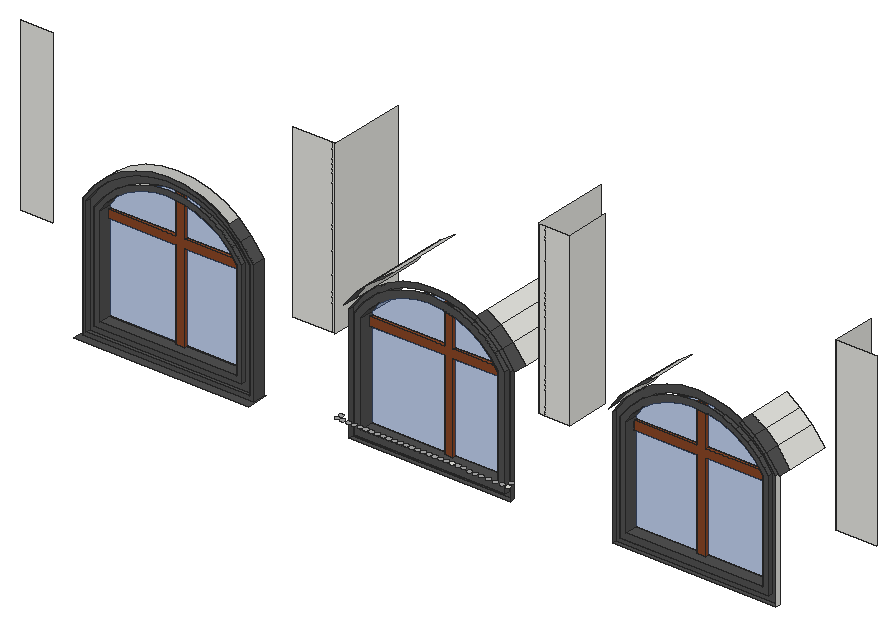
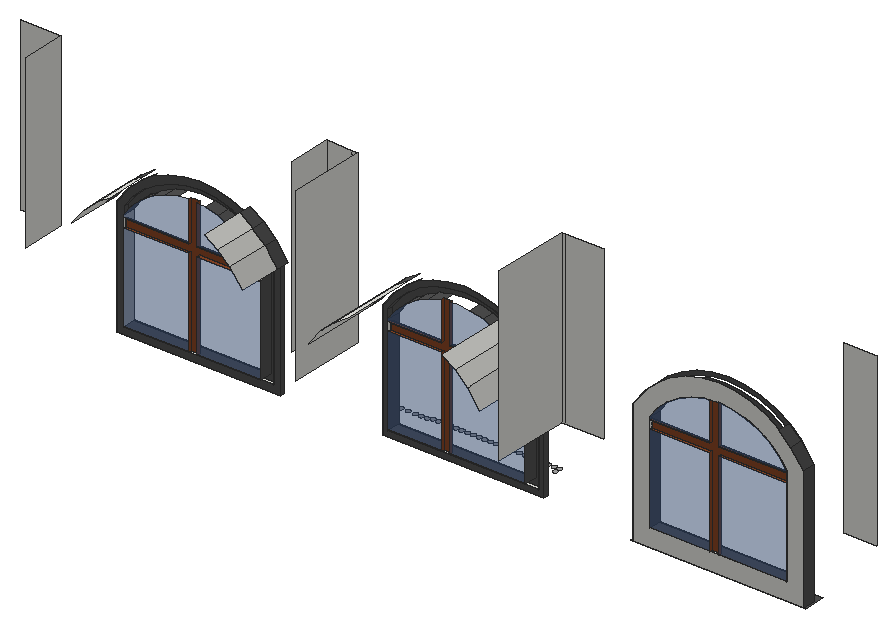
# SketchUp Ruby script. Lengths in inches.
U = 1.inch
M = Sketchup.active_model
def pt(a) = Geom::Point3d.new(a.map { |v| v * U })
def face(e, loops, mat)
  f = e.add_face(loops[0].map { |a| pt(a) })
  loops[1..].each { |l| e.add_face(l.map { |a| pt(a) }).erase! }
  f.material = f.back_material = mat if mat
  f
end
# faces: each face lists its corners as indices into pts; further lists are holes
def faces(e, pts, list, mat = nil) = list.each { |f| face(e, (f[0].is_a?(Array) ? f : [f]).map { |l| l.map { |i| pts[i] } }, mat) }
# xy, xz, yz: faces in a plane at the given z, y or x. An outline is a flat list of corners, or four numbers for a rectangle; further outlines are holes
def ring(l) = l.size == 4 ? [[l[0], l[1]], [l[2], l[1]], [l[2], l[3]], [l[0], l[3]]] : l.each_slice(2).to_a
def flat(e, list, mat, &to3) = list.each { |f| face(e, (f[0].is_a?(Array) ? f : [f]).map { |l| ring(l).map { |u, v| to3.(u, v) } }, mat) }
def xy(e, z, list, mat = nil) = flat(e, list, mat) { |x, y| [x, y, z] }
def xz(e, y, list, mat = nil) = flat(e, list, mat) { |x, z| [x, y, z] }
def yz(e, x, list, mat = nil) = flat(e, list, mat) { |y, z| [x, y, z] }
def lines(e, pts, list) = list.each { |a, b| e.add_line(pt(pts[a]), pt(pts[b])) }
# prism: a flat outline (further loops are holes) pulled along v
def prism(e, loops, v, mat = nil)
  f = face(e, loops, mat); d = Geom::Vector3d.new(v.map { |x| x * U })
  f.pushpull(f.normal.samedirection?(d) ? d.length : -d.length)
end
def box(e, o, s, mat = nil) = prism(e, [[o, [o[0] + s[0], o[1], o[2]], [o[0] + s[0], o[1] + s[1], o[2]], [o[0], o[1] + s[1], o[2]]]], [0, 0, s[2]], mat)
def at(x, y, z, deg = 0) = Geom::Transformation.translation(pt([x, y, z])) * Geom::Transformation.rotation(ORIGIN, Z_AXIS, deg.degrees)
def axes(o, x, y, z) = Geom::Transformation.new([*x, 0, *y, 0, *z, 0, *pt(o).to_a, 1])
def part(name) = M.definitions.add(name)
# library, detail: a bought-in or finely detailed component or shape, given as its bounding box
def library(name, o, s) = part(name).tap { |d| box(d.entities, o, s) }
def detail(e, o, s) = box(e.add_group.entities, o, s)
def put(e, d, t, mat = nil) = e.add_instance(d, t).tap { |i| i.material = mat if mat }
def group(e, t, mat = nil) = e.add_group.tap { |g| g.transformation = t; g.material = mat if mat }.entities
root = M.entities
M.materials.add("[0042_Sienna]").color = [137, 70, 38]
M.materials.add("[0132_LightGray]").color = [169, 169, 169]
M.materials.add("[0135_DarkGray]").color = [81, 81, 81]
M.materials.add("[Translucent Glass Blue]").color = [66, 99, 158]
M.materials["[Translucent Glass Blue]"].alpha = 0.5
xy(root,182.98,[[429.64,40.6875,544.9375,43.6875]],"[0135_DarkGray]")
xy(root,183.1,[[55.95,40.6875,176.64,49.6875]])
xy(root,183.1,[[54.57,34.6875,177.76,34.6875,177.76,49.6875,176.64,49.6875,176.64,40.6875,55.95,40.6875,55.95,49.6875,54.57,49.6875]],"[0135_DarkGray]")
xy(root,183.73,[[243.9,40.6875,357.68,43.6875]],"[0135_DarkGray]")
xy(root,185.78,[[58.63,40.6875,173.95,43.6875]],"[0135_DarkGray]")
xy(root,187.34,[[247.51,40.6875,354.08,43.6875]])
xy(root,188.0625,[[434.73,40.6875,539.86,43.6875]])
xy(root,191.43,[[64.29,40.6875,168.3,43.6875]],"[0135_DarkGray]")
xy(root,192.28,[[305.64,47.6875,311.64,49.6875],[483.7,47.6875,489.7,49.6875]])
xy(root,192.28,[[252.45,40.6875,349.14,40.6875,349.14,49.6875,311.64,49.6875,311.64,47.6875,305.64,47.6875,305.64,49.6875,252.45,49.6875],[438.95,40.6875,535.64,40.6875,535.64,49.6875,489.7,49.6875,489.7,47.6875,483.7,47.6875,483.7,49.6875,438.95,49.6875]],"[0135_DarkGray]")
xy(root,195.1,[[116.29,47.6875,122.29,49.6875]])
xy(root,195.1,[[67.95,40.6875,164.64,40.6875,164.64,49.6875,122.29,49.6875,122.29,47.6875,116.29,47.6875,116.29,49.6875,67.95,49.6875]],"[0135_DarkGray]")
xy(root,197.66,[[361.68,32.09,362.06,32.13,362.4,32.28,362.7,32.51,362.93,32.8,363.07,33.15,363.12,33.52,363.07,33.89,362.93,34.24,362.7,34.54,362.4,34.77,362.06,34.91,361.68,34.96,361.3125,34.91,360.97,34.77,360.67,34.54,360.4375,34.24,360.3,33.89,360.25,33.52,360.3,33.15,360.4375,32.8,360.67,32.51,360.97,32.28,361.3125,32.13]])
xy(root,197.66,[[334.56,32.09,334.93,32.13,335.28,32.28,335.58,32.51,335.8,32.8,335.95,33.15,336,33.52,335.95,33.89,335.8,34.24,335.58,34.54,335.28,34.77,334.93,34.91,334.56,34.96,334.1875,34.91,333.84,34.77,333.54,34.54,333.3125,34.24,333.17,33.89,333.12,33.52,333.17,33.15,333.3125,32.8,333.54,32.51,333.84,32.28,334.1875,32.13],[338.62,32.09,338.99,32.13,339.34,32.28,339.64,32.51,339.87,32.8,340.01,33.15,340.06,33.52,340.01,33.89,339.87,34.24,339.64,34.54,339.34,34.77,338.99,34.91,338.62,34.96,338.25,34.91,337.9,34.77,337.6,34.54,337.375,34.24,337.23,33.89,337.18,33.52,337.23,33.15,337.375,32.8,337.6,32.51,337.9,32.28,338.25,32.13],[342.68,32.09,343.06,32.13,343.4,32.28,343.7,32.51,343.93,32.8,344.07,33.15,344.12,33.52,344.07,33.89,343.93,34.24,343.7,34.54,343.4,34.77,343.06,34.91,342.68,34.96,342.3125,34.91,341.97,34.77,341.67,34.54,341.4375,34.24,341.3,33.89,341.25,33.52,341.3,33.15,341.4375,32.8,341.67,32.51,341.97,32.28,342.3125,32.13],[347.93,32.09,348.31,32.13,348.65,32.28,348.95,32.51,349.18,32.8,349.32,33.15,349.37,33.52,349.32,33.89,349.18,34.24,348.95,34.54,348.65,34.77,348.31,34.91,347.93,34.96,347.5625,34.91,347.22,34.77,346.92,34.54,346.6875,34.24,346.55,33.89,346.5,33.52,346.55,33.15,346.6875,32.8,346.92,32.51,347.22,32.28,347.5625,32.13],[352.81,32.09,353.18,32.13,353.53,32.28,353.83,32.51,354.05,32.8,354.2,33.15,354.25,33.52,354.2,33.89,354.05,34.24,353.83,34.54,353.53,34.77,353.18,34.91,352.81,34.96,352.4375,34.91,352.09,34.77,351.79,34.54,351.5625,34.24,351.42,33.89,351.37,33.52,351.42,33.15,351.5625,32.8,351.79,32.51,352.09,32.28,352.4375,32.13],
  [357.56,32.09,357.93,32.13,358.28,32.28,358.58,32.51,358.8,32.8,358.95,33.15,359,33.52,358.95,33.89,358.8,34.24,358.58,34.54,358.28,34.77,357.93,34.91,357.56,34.96,357.1875,34.91,356.84,34.77,356.54,34.54,356.3125,34.24,356.17,33.89,356.12,33.52,356.17,33.15,356.3125,32.8,356.54,32.51,356.84,32.28,357.1875,32.13],[360.7,36.35,361.07,36.4,361.41,36.54,361.71,36.77,361.94,37.07,362.08,37.41,362.13,37.78,362.08,38.16,361.94,38.5,361.71,38.8,361.41,39.03,361.07,39.17,360.7,39.22,360.32,39.17,359.98,39.03,359.68,38.8,359.45,38.5,359.31,38.16,359.26,37.78,359.31,37.41,359.45,37.07,359.68,36.77,359.98,36.54,360.32,36.4]],"[0132_LightGray]")
xy(root,198.6,[[322.37,32.09,322.74,32.13,323.09,32.28,323.39,32.51,323.62,32.8,323.76,33.15,323.81,33.52,323.76,33.89,323.62,34.24,323.39,34.54,323.09,34.77,322.74,34.91,322.37,34.96,322,34.91,321.65,34.77,321.35,34.54,321.125,34.24,320.98,33.89,320.93,33.52,320.98,33.15,321.125,32.8,321.35,32.51,321.65,32.28,322,32.13]])
xy(root,198.6,[[241.12,32.09,241.49,32.13,241.84,32.28,242.14,32.51,242.37,32.8,242.51,33.15,242.56,33.52,242.51,33.89,242.37,34.24,242.14,34.54,241.84,34.77,241.49,34.91,241.12,34.96,240.75,34.91,240.4,34.77,240.1,34.54,239.875,34.24,239.73,33.89,239.68,33.52,239.73,33.15,239.875,32.8,240.1,32.51,240.4,32.28,240.75,32.13],[245.18,32.09,245.56,32.13,245.9,32.28,246.2,32.51,246.43,32.8,246.57,33.15,246.62,33.52,246.57,33.89,246.43,34.24,246.2,34.54,245.9,34.77,245.56,34.91,245.18,34.96,244.8125,34.91,244.47,34.77,244.17,34.54,243.9375,34.24,243.8,33.89,243.75,33.52,243.8,33.15,243.9375,32.8,244.17,32.51,244.47,32.28,244.8125,32.13],[249.25,32.09,249.62,32.13,249.97,32.28,250.26,32.51,250.49,32.8,250.63,33.15,250.68,33.52,250.63,33.89,250.49,34.24,250.26,34.54,249.97,34.77,249.62,34.91,249.25,34.96,248.875,34.91,248.53,34.77,248.23,34.54,248,34.24,247.86,33.89,247.81,33.52,247.86,33.15,248,32.8,248.23,32.51,248.53,32.28,248.875,32.13],[253.31,32.09,253.68,32.13,254.03,32.28,254.33,32.51,254.55,32.8,254.7,33.15,254.75,33.52,254.7,33.89,254.55,34.24,254.33,34.54,254.03,34.77,253.68,34.91,253.31,34.96,252.9375,34.91,252.59,34.77,252.29,34.54,252.0625,34.24,251.92,33.89,251.87,33.52,251.92,33.15,252.0625,32.8,252.29,32.51,252.59,32.28,252.9375,32.13],[257.37,32.09,257.74,32.13,258.09,32.28,258.39,32.51,258.62,32.8,258.76,33.15,258.81,33.52,258.76,33.89,258.62,34.24,258.39,34.54,258.09,34.77,257.74,34.91,257.37,34.96,257,34.91,256.65,34.77,256.35,34.54,256.125,34.24,255.98,33.89,255.93,33.52,255.98,33.15,256.125,32.8,256.35,32.51,256.65,32.28,257,32.13],
  [261.43,32.09,261.81,32.13,262.15,32.28,262.45,32.51,262.68,32.8,262.82,33.15,262.87,33.52,262.82,33.89,262.68,34.24,262.45,34.54,262.15,34.77,261.81,34.91,261.43,34.96,261.0625,34.91,260.72,34.77,260.42,34.54,260.1875,34.24,260.05,33.89,260,33.52,260.05,33.15,260.1875,32.8,260.42,32.51,260.72,32.28,261.0625,32.13],[265.5,32.09,265.87,32.13,266.22,32.28,266.51,32.51,266.74,32.8,266.88,33.15,266.93,33.52,266.88,33.89,266.74,34.24,266.51,34.54,266.22,34.77,265.87,34.91,265.5,34.96,265.125,34.91,264.78,34.77,264.48,34.54,264.25,34.24,264.11,33.89,264.06,33.52,264.11,33.15,264.25,32.8,264.48,32.51,264.78,32.28,265.125,32.13],[269.56,32.09,269.93,32.13,270.28,32.28,270.58,32.51,270.8,32.8,270.95,33.15,271,33.52,270.95,33.89,270.8,34.24,270.58,34.54,270.28,34.77,269.93,34.91,269.56,34.96,269.1875,34.91,268.84,34.77,268.54,34.54,268.3125,34.24,268.17,33.89,268.12,33.52,268.17,33.15,268.3125,32.8,268.54,32.51,268.84,32.28,269.1875,32.13],[273.62,32.09,273.99,32.13,274.34,32.28,274.64,32.51,274.87,32.8,275.01,33.15,275.06,33.52,275.01,33.89,274.87,34.24,274.64,34.54,274.34,34.77,273.99,34.91,273.62,34.96,273.25,34.91,272.9,34.77,272.6,34.54,272.375,34.24,272.23,33.89,272.18,33.52,272.23,33.15,272.375,32.8,272.6,32.51,272.9,32.28,273.25,32.13],[277.68,32.09,278.06,32.13,278.4,32.28,278.7,32.51,278.93,32.8,279.07,33.15,279.12,33.52,279.07,33.89,278.93,34.24,278.7,34.54,278.4,34.77,278.06,34.91,277.68,34.96,277.3125,34.91,276.97,34.77,276.67,34.54,276.4375,34.24,276.3,33.89,276.25,33.52,276.3,33.15,276.4375,32.8,276.67,32.51,276.97,32.28,277.3125,32.13],
  [281.75,32.09,282.12,32.13,282.47,32.28,282.76,32.51,282.99,32.8,283.13,33.15,283.18,33.52,283.13,33.89,282.99,34.24,282.76,34.54,282.47,34.77,282.12,34.91,281.75,34.96,281.375,34.91,281.03,34.77,280.73,34.54,280.5,34.24,280.36,33.89,280.31,33.52,280.36,33.15,280.5,32.8,280.73,32.51,281.03,32.28,281.375,32.13],[285.81,32.09,286.18,32.13,286.53,32.28,286.83,32.51,287.05,32.8,287.2,33.15,287.25,33.52,287.2,33.89,287.05,34.24,286.83,34.54,286.53,34.77,286.18,34.91,285.81,34.96,285.4375,34.91,285.09,34.77,284.79,34.54,284.5625,34.24,284.42,33.89,284.37,33.52,284.42,33.15,284.5625,32.8,284.79,32.51,285.09,32.28,285.4375,32.13],[289.87,32.09,290.24,32.13,290.59,32.28,290.89,32.51,291.12,32.8,291.26,33.15,291.31,33.52,291.26,33.89,291.12,34.24,290.89,34.54,290.59,34.77,290.24,34.91,289.87,34.96,289.5,34.91,289.15,34.77,288.85,34.54,288.625,34.24,288.48,33.89,288.43,33.52,288.48,33.15,288.625,32.8,288.85,32.51,289.15,32.28,289.5,32.13],[293.93,32.09,294.31,32.13,294.65,32.28,294.95,32.51,295.18,32.8,295.32,33.15,295.37,33.52,295.32,33.89,295.18,34.24,294.95,34.54,294.65,34.77,294.31,34.91,293.93,34.96,293.5625,34.91,293.22,34.77,292.92,34.54,292.6875,34.24,292.55,33.89,292.5,33.52,292.55,33.15,292.6875,32.8,292.92,32.51,293.22,32.28,293.5625,32.13],[298,32.09,298.37,32.13,298.72,32.28,299.01,32.51,299.24,32.8,299.38,33.15,299.43,33.52,299.38,33.89,299.24,34.24,299.01,34.54,298.72,34.77,298.37,34.91,298,34.96,297.625,34.91,297.28,34.77,296.98,34.54,296.75,34.24,296.61,33.89,296.56,33.52,296.61,33.15,296.75,32.8,296.98,32.51,297.28,32.28,297.625,32.13],
  [302.06,32.09,302.43,32.13,302.78,32.28,303.08,32.51,303.3,32.8,303.45,33.15,303.5,33.52,303.45,33.89,303.3,34.24,303.08,34.54,302.78,34.77,302.43,34.91,302.06,34.96,301.6875,34.91,301.34,34.77,301.04,34.54,300.8125,34.24,300.67,33.89,300.62,33.52,300.67,33.15,300.8125,32.8,301.04,32.51,301.34,32.28,301.6875,32.13],[306.12,32.09,306.49,32.13,306.84,32.28,307.14,32.51,307.37,32.8,307.51,33.15,307.56,33.52,307.51,33.89,307.37,34.24,307.14,34.54,306.84,34.77,306.49,34.91,306.12,34.96,305.75,34.91,305.4,34.77,305.1,34.54,304.875,34.24,304.73,33.89,304.68,33.52,304.73,33.15,304.875,32.8,305.1,32.51,305.4,32.28,305.75,32.13],[310.18,32.09,310.56,32.13,310.9,32.28,311.2,32.51,311.43,32.8,311.57,33.15,311.62,33.52,311.57,33.89,311.43,34.24,311.2,34.54,310.9,34.77,310.56,34.91,310.18,34.96,309.8125,34.91,309.47,34.77,309.17,34.54,308.9375,34.24,308.8,33.89,308.75,33.52,308.8,33.15,308.9375,32.8,309.17,32.51,309.47,32.28,309.8125,32.13],[314.25,32.09,314.62,32.13,314.97,32.28,315.26,32.51,315.49,32.8,315.63,33.15,315.68,33.52,315.63,33.89,315.49,34.24,315.26,34.54,314.97,34.77,314.62,34.91,314.25,34.96,313.875,34.91,313.53,34.77,313.23,34.54,313,34.24,312.86,33.89,312.81,33.52,312.86,33.15,313,32.8,313.23,32.51,313.53,32.28,313.875,32.13],[318.31,32.09,318.68,32.13,319.03,32.28,319.33,32.51,319.55,32.8,319.7,33.15,319.75,33.52,319.7,33.89,319.55,34.24,319.33,34.54,319.03,34.77,318.68,34.91,318.31,34.96,317.9375,34.91,317.59,34.77,317.29,34.54,317.0625,34.24,316.92,33.89,316.87,33.52,316.92,33.15,317.0625,32.8,317.29,32.51,317.59,32.28,317.9375,32.13],
  [326.43,32.09,326.81,32.13,327.15,32.28,327.45,32.51,327.68,32.8,327.82,33.15,327.87,33.52,327.82,33.89,327.68,34.24,327.45,34.54,327.15,34.77,326.81,34.91,326.43,34.96,326.0625,34.91,325.72,34.77,325.42,34.54,325.1875,34.24,325.05,33.89,325,33.52,325.05,33.15,325.1875,32.8,325.42,32.51,325.72,32.28,326.0625,32.13],[330.5,32.09,330.87,32.13,331.22,32.28,331.51,32.51,331.74,32.8,331.88,33.15,331.93,33.52,331.88,33.89,331.74,34.24,331.51,34.54,331.22,34.77,330.87,34.91,330.5,34.96,330.125,34.91,329.78,34.77,329.48,34.54,329.25,34.24,329.11,33.89,329.06,33.52,329.11,33.15,329.25,32.8,329.48,32.51,329.78,32.28,330.125,32.13],[241.12,35.71,241.49,35.76,241.84,35.9,242.14,36.13,242.37,36.43,242.51,36.78,242.56,37.15,242.51,37.52,242.37,37.87,242.14,38.16,241.84,38.39,241.49,38.54,241.12,38.59,240.75,38.54,240.4,38.39,240.1,38.16,239.875,37.87,239.73,37.52,239.68,37.15,239.73,36.78,239.875,36.43,240.1,36.13,240.4,35.9,240.75,35.76]],"[0132_LightGray]")
xy(root,254.53,[[438.95,47.6875,483.7,49.6875],[489.7,47.6875,535.64,49.6875]],"[0042_Sienna]")
xy(root,254.85,[[252.45,47.6875,305.64,49.6875],[311.64,47.6875,349.14,49.6875]],"[0042_Sienna]")
xy(root,257.72,[[67.95,47.6875,116.29,49.6875],[122.29,47.6875,164.64,49.6875]],"[0042_Sienna]")
xy(root,260.53,[[438.95,47.6875,483.7,49.6875],[489.7,47.6875,535.64,49.6875]],"[0042_Sienna]")
xy(root,260.85,[[252.45,47.6875,305.64,49.6875],[311.64,47.6875,349.14,49.6875]],"[0042_Sienna]")
xy(root,263.72,[[67.95,47.6875,116.29,49.6875],[122.29,47.6875,164.64,49.6875]],"[0042_Sienna]")
xz(root,40.6875,[[[55.95,183.1,176.64,183.1,176.64,269.51,167.71,281.11,159.24,288.98,149.59,295.34,139.01,300.01,127.8125,302.86,116.29,303.82,104.77,302.86,93.57,300.01,83,295.34,73.34,288.98,64.875,281.11,55.95,269.51],[58.63,185.78,58.63,268.6,66.87,279.3,75.01,286.86,84.29,292.97,94.45,297.46,105.22,300.21,116.29,301.13,127.36,300.21,138.13,297.46,148.3,292.97,157.58,286.86,165.72,279.3,173.95,268.6,173.95,185.78]],[[247.51,187.34,354.08,187.34,354.08,264.3,346.97,273.53,339.37,280.6,330.7,286.31,321.2,290.5,311.14,293.07,300.79,293.93,290.44,293.07,280.38,290.5,270.89,286.31,262.22,280.6,254.61,273.53,247.51,264.3],[252.45,192.28,252.45,262.62,258.28,270.19,265.28,276.7,273.26,281.95,282,285.82,291.27,288.18,300.79,288.97,310.32,288.18,319.58,285.82,328.32,281.95,336.3,276.7,343.31,270.19,349.14,262.62,349.14,192.28]],[[434.73,188.0625,539.86,188.0625,539.86,264.05,532.9375,273.04,525.42,280.03,516.85,285.67,507.46,289.82,497.52,292.35,487.29,293.21,477.06,292.35,467.12,289.82,457.73,285.67,449.16,280.03,441.64,273.04,434.73,264.05],[438.95,192.28,438.95,262.62,444.78,270.19,451.78,276.7,459.76,281.95,468.5,285.82,477.77,288.18,487.29,288.97,496.82,288.18,506.08,285.82,514.82,281.95,522.8,276.7,529.81,270.19,535.64,262.62,535.64,192.28]],[[64.29,191.43,168.3,191.43,168.3,266.67,161.52,275.48,154.07,282.4,145.58,287.99,136.28,292.1,126.42,294.61,116.29,295.46,106.16,294.61,96.3,292.1,87,287.99,78.51,282.4,71.06,275.48,64.29,266.67],[67.95,195.1,67.95,265.43,73.78,273,80.78,279.51,88.76,284.77,97.5,288.63,106.77,290.99,116.29,291.78,125.82,290.99,135.08,288.63,143.82,284.77,151.8,279.51,158.81,273,164.64,265.43,164.64,195.1]]],"[0135_DarkGray]")
xz(root,43.6875,[[[429.64,182.98,544.9375,182.98,544.9375,265.78,536.71,276.48,528.57,284.04,519.29,290.15,509.13,294.64,498.36,297.38,487.29,298.31,476.22,297.38,465.45,294.64,455.29,290.15,446.01,284.04,437.875,276.48,429.64,265.78],[434.73,188.0625,434.73,264.05,441.64,273.04,449.16,280.03,457.73,285.67,467.12,289.82,477.06,292.35,487.29,293.21,497.52,292.35,507.46,289.82,516.85,285.67,525.42,280.03,532.9375,273.04,539.86,264.05,539.86,188.0625]],[[243.9,183.73,357.68,183.73,357.68,265.52,349.65,275.97,341.6,283.44,332.43,289.48,322.38,293.92,311.74,296.64,300.79,297.55,289.85,296.64,279.2,293.92,269.16,289.48,259.98,283.44,251.94,275.97,243.9,265.52],[247.51,187.34,247.51,264.3,254.61,273.53,262.22,280.6,270.89,286.31,280.38,290.5,290.44,293.07,300.79,293.93,311.14,293.07,321.2,290.5,330.7,286.31,339.37,280.6,346.97,273.53,354.08,264.3,354.08,187.34]],[[58.63,185.78,173.95,185.78,173.95,268.6,165.72,279.3,157.58,286.86,148.3,292.97,138.13,297.46,127.36,300.21,116.29,301.13,105.22,300.21,94.45,297.46,84.29,292.97,75.01,286.86,66.87,279.3,58.63,268.6],[64.29,191.43,64.29,266.67,71.06,275.48,78.51,282.4,87,287.99,96.3,292.1,106.16,294.61,116.29,295.46,126.42,294.61,136.28,292.1,145.58,287.99,154.07,282.4,161.52,275.48,168.3,266.67,168.3,191.43]]],"[0135_DarkGray]")
xz(root,47.6875,[[305.64,192.28,311.64,192.28,311.64,254.85,349.14,254.85,349.14,260.85,311.64,260.85,311.64,287.84,310.32,288.18,305.64,288.57,305.64,260.85,252.45,260.85,252.45,254.85,305.64,254.85],[483.7,192.28,489.7,192.28,489.7,254.53,535.64,254.53,535.64,260.53,489.7,260.53,489.7,288.77,487.29,288.97,483.7,288.67,483.7,260.53,438.95,260.53,438.95,254.53,483.7,254.53],[116.29,195.1,122.29,195.1,122.29,257.72,164.64,257.72,164.64,263.72,122.29,263.72,122.29,291.28,116.29,291.78,116.29,263.72,67.95,263.72,67.95,257.72,116.29,257.72]],"[0042_Sienna]")
xz(root,49.6875,[[[55.95,183.1,176.64,183.1,176.64,269.51,167.71,281.11,159.24,288.98,149.59,295.34,139.01,300.01,127.8125,302.86,116.29,303.82,104.77,302.86,93.57,300.01,83,295.34,73.34,288.98,64.875,281.11,55.95,269.51],[67.95,195.1,67.95,265.43,73.78,273,80.78,279.51,88.76,284.77,97.5,288.63,106.77,290.99,116.29,291.78,122.29,291.28,125.82,290.99,135.08,288.63,143.82,284.77,151.8,279.51,158.81,273,164.64,265.43,164.64,195.1]],[4.9375,240,27.68,360],[197.35,240,224.47,360],[224.47,240,226.6,360],[226.6,240,227.04,360],
  [370.55,240,370.74,360],[370.74,240,374.55,360],[374.55,240,392.7,360],[580.01,240,608.5,360]])
xz(root,49.6875,[[252.45,192.28,305.64,254.85],[311.64,192.28,349.14,254.85],[438.95,192.28,483.7,254.53],[489.7,192.28,535.64,254.53],[67.95,195.1,116.29,257.72],
  [122.29,195.1,164.64,257.72],[438.95,260.53,483.7,260.53,483.7,288.67,477.77,288.18,468.5,285.82,459.76,281.95,451.78,276.7,444.78,270.19,438.95,262.62],[489.7,260.53,535.64,260.53,535.64,262.62,529.81,270.19,522.8,276.7,514.82,281.95,506.08,285.82,496.82,288.18,489.7,288.77],[252.45,260.85,305.64,260.85,305.64,288.57,300.79,288.97,291.27,288.18,282,285.82,273.26,281.95,265.28,276.7,258.28,270.19,252.45,262.62],[311.64,260.85,349.14,260.85,349.14,262.62,343.31,270.19,336.3,276.7,328.32,281.95,319.58,285.82,311.64,287.84],
  [67.95,263.72,116.29,263.72,116.29,291.78,106.77,290.99,97.5,288.63,88.76,284.77,80.78,279.51,73.78,273,67.95,265.43],[122.29,263.72,164.64,263.72,164.64,265.43,158.81,273,151.8,279.51,143.82,284.77,135.08,288.63,125.82,290.99,122.29,291.28]],"[Translucent Glass Blue]")
yz(root,55.95,[[40.6875,183.1,49.6875,269.51]],"[0135_DarkGray]")
yz(root,58.63,[[40.6875,185.78,43.6875,268.6]],"[0135_DarkGray]")
yz(root,64.29,[[40.6875,191.43,43.6875,266.67]],"[0135_DarkGray]")
yz(root,67.95,[[47.6875,257.72,49.6875,263.72]])
yz(root,67.95,[[40.6875,195.1,49.6875,195.1,49.6875,257.72,47.6875,257.72,47.6875,263.72,49.6875,263.72,49.6875,265.43,40.6875,265.43]],"[0135_DarkGray]")
yz(root,116.29,[[47.6875,195.1,49.6875,257.72],[47.6875,263.72,49.6875,291.78]],"[0042_Sienna]")
yz(root,122.29,[[47.6875,195.1,49.6875,257.72],[47.6875,263.72,49.6875,291.28]],"[0042_Sienna]")
yz(root,164.64,[[47.6875,257.72,49.6875,263.72]])
yz(root,164.64,[[40.6875,195.1,40.6875,265.43,49.6875,265.43,49.6875,263.72,47.6875,263.72,47.6875,257.72,49.6875,257.72,49.6875,195.1]],"[0135_DarkGray]")
yz(root,168.3,[[40.6875,191.43,43.6875,266.67]],"[0135_DarkGray]")
yz(root,173.95,[[40.6875,185.78,43.6875,268.6]],"[0135_DarkGray]")
yz(root,176.64,[[40.6875,183.1,49.6875,269.51]],"[0135_DarkGray]")
yz(root,227.04,[[49.6875,240,104.375,360]])
yz(root,243.9,[[40.6875,183.73,43.6875,265.52]],"[0135_DarkGray]")
yz(root,247.51,[[40.6875,187.34,43.6875,264.3]],"[0135_DarkGray]")
yz(root,252.45,[[47.6875,254.85,49.6875,260.85]])
yz(root,252.45,[[40.6875,192.28,49.6875,192.28,49.6875,254.85,47.6875,254.85,47.6875,260.85,49.6875,260.85,49.6875,262.62,40.6875,262.62]],"[0135_DarkGray]")
yz(root,305.64,[[47.6875,192.28,49.6875,254.85],[47.6875,260.85,49.6875,288.57]],"[0042_Sienna]")
yz(root,311.64,[[47.6875,192.28,49.6875,254.85],[47.6875,260.85,49.6875,287.84]],"[0042_Sienna]")
yz(root,349.14,[[47.6875,254.85,49.6875,260.85]])
yz(root,349.14,[[40.6875,192.28,40.6875,262.62,49.6875,262.62,49.6875,260.85,47.6875,260.85,47.6875,254.85,49.6875,254.85,49.6875,192.28]],"[0135_DarkGray]")
yz(root,354.08,[[40.6875,187.34,43.6875,264.3]],"[0135_DarkGray]")
yz(root,357.68,[[40.6875,183.73,43.6875,265.52]],"[0135_DarkGray]")
yz(root,370.55,[[49.6875,240,104.375,360]])
yz(root,392.7,[[49.6875,240,80.4375,360]])
yz(root,429.64,[[40.6875,182.98,43.6875,265.78]],"[0135_DarkGray]")
yz(root,434.73,[[40.6875,188.0625,43.6875,264.05]])
yz(root,438.95,[[47.6875,254.53,49.6875,260.53]])
yz(root,438.95,[[40.6875,192.28,49.6875,192.28,49.6875,254.53,47.6875,254.53,47.6875,260.53,49.6875,260.53,49.6875,262.62,40.6875,262.62]],"[0135_DarkGray]")
yz(root,483.7,[[47.6875,192.28,49.6875,254.53],[47.6875,260.53,49.6875,288.67]],"[0042_Sienna]")
yz(root,489.7,[[47.6875,192.28,49.6875,254.53],[47.6875,260.53,49.6875,288.77]],"[0042_Sienna]")
yz(root,535.64,[[40.6875,192.28,40.6875,262.62,49.6875,262.62,49.6875,260.53,47.6875,260.53,47.6875,254.53,49.6875,254.53,49.6875,192.28],[47.6875,254.53,49.6875,260.53]])
yz(root,539.86,[[40.6875,188.0625,43.6875,264.05]],"[0135_DarkGray]")
yz(root,544.9375,[[40.6875,182.98,43.6875,265.78]])
yz(root,580.01,[[49.6875,240,80.4375,360]])
p = [[252.45,49.6875,262.62],[258.28,49.6875,270.19],[258.28,40.6875,270.19],[252.45,40.6875,262.62],[343.31,49.6875,270.19],[349.14,49.6875,262.62],
  [349.14,40.6875,262.62],[343.31,40.6875,270.19],[438.95,49.6875,262.62],[444.78,49.6875,270.19],[444.78,40.6875,270.19],[438.95,40.6875,262.62],
  [529.81,49.6875,270.19],[535.64,49.6875,262.62],[535.64,40.6875,262.62],[529.81,40.6875,270.19],[441.64,43.6875,273.04],[434.73,43.6875,264.05],
  [434.73,40.6875,264.05],[441.64,40.6875,273.04],[539.86,43.6875,264.05],[532.9375,43.6875,273.04],[532.9375,40.6875,273.04],[539.86,40.6875,264.05],
  [254.61,43.6875,273.53],[247.51,43.6875,264.3],[247.51,40.6875,264.3],[254.61,40.6875,273.53],[354.08,43.6875,264.3],[346.97,43.6875,273.53],
  [346.97,40.6875,273.53],[354.08,40.6875,264.3],[67.95,49.6875,265.43],[73.78,49.6875,273],[73.78,40.6875,273],[67.95,40.6875,265.43],
  [158.81,49.6875,273],[164.64,49.6875,265.43],[164.64,40.6875,265.43],[158.81,40.6875,273],[243.9,43.6875,265.52],[251.94,43.6875,275.97],
  [251.94,40.6875,275.97],[243.9,40.6875,265.52],[349.65,43.6875,275.97],[357.68,43.6875,265.52],[357.68,40.6875,265.52],[349.65,40.6875,275.97],
  [429.64,43.6875,265.78],[437.875,43.6875,276.48],[437.875,40.6875,276.48],[429.64,40.6875,265.78],[536.71,43.6875,276.48],[544.9375,43.6875,265.78],
  [544.9375,40.6875,265.78],[536.71,40.6875,276.48],[71.06,43.6875,275.48],[64.29,43.6875,266.67],[64.29,40.6875,266.67],[71.06,40.6875,275.48],
  [168.3,43.6875,266.67],[161.52,43.6875,275.48],[161.52,40.6875,275.48],[168.3,40.6875,266.67],[249.375,49.6875,278.3],[240.45,49.6875,266.7],
  [240.45,40.6875,266.7],[249.375,40.6875,278.3],[361.14,49.6875,266.7],[352.21,49.6875,278.3],[352.21,40.6875,278.3],[361.14,40.6875,266.7],
  [426.95,49.6875,266.7],[435.875,49.6875,278.3],[435.875,40.6875,278.3],[426.95,40.6875,266.7],[538.71,49.6875,278.3],[547.64,49.6875,266.7],
  [547.64,40.6875,266.7],[538.71,40.6875,278.3],[240.45,104.375,266.7],[249.375,104.375,278.3],[352.21,104.375,278.3],[361.14,104.375,266.7],
  [426.95,80.4375,266.7],[435.875,80.4375,278.3],[538.71,80.4375,278.3],[547.64,80.4375,266.7],[58.63,43.6875,268.6],[66.87,43.6875,279.3],
  [66.87,40.6875,279.3],[58.63,40.6875,268.6],[165.72,43.6875,279.3],[173.95,43.6875,268.6],[173.95,40.6875,268.6],[165.72,40.6875,279.3],
  [64.875,49.6875,281.11],[55.95,49.6875,269.51],[55.95,40.6875,269.51],[64.875,40.6875,281.11],[176.64,49.6875,269.51],[167.71,49.6875,281.11],
  [167.71,40.6875,281.11],[176.64,40.6875,269.51],[265.28,49.6875,276.7],[265.28,40.6875,276.7],[336.3,49.6875,276.7],[336.3,40.6875,276.7],
  [451.78,49.6875,276.7],[451.78,40.6875,276.7],[522.8,49.6875,276.7],[522.8,40.6875,276.7],[80.78,49.6875,279.51],[80.78,40.6875,279.51],
  [151.8,49.6875,279.51],[151.8,40.6875,279.51],[449.16,43.6875,280.03],[449.16,40.6875,280.03],[525.42,43.6875,280.03],[525.42,40.6875,280.03],
  [262.22,43.6875,280.6],[262.22,40.6875,280.6],[339.37,43.6875,280.6],[339.37,40.6875,280.6],[78.51,43.6875,282.4],[78.51,40.6875,282.4],
  [154.07,43.6875,282.4],[154.07,40.6875,282.4],[259.98,43.6875,283.44],[259.98,40.6875,283.44],[341.6,43.6875,283.44],[341.6,40.6875,283.44],
  [446.01,43.6875,284.04],[446.01,40.6875,284.04],[528.57,43.6875,284.04],[528.57,40.6875,284.04],[273.26,49.6875,281.95],[273.26,40.6875,281.95],
  [328.32,49.6875,281.95],[328.32,40.6875,281.95],[459.76,49.6875,281.95],[459.76,40.6875,281.95],[514.82,49.6875,281.95],[514.82,40.6875,281.95],
  [257.84,49.6875,286.17],[257.84,40.6875,286.17],[343.74,49.6875,286.17],[343.74,40.6875,286.17],[444.34,49.6875,286.17],[444.34,40.6875,286.17],
  [530.24,49.6875,286.17],[530.24,40.6875,286.17],[257.84,104.375,286.17],[343.74,104.375,286.17],[444.34,80.4375,286.17],[530.24,80.4375,286.17],
  [75.01,43.6875,286.86],[75.01,40.6875,286.86],[157.58,43.6875,286.86],[157.58,40.6875,286.86],[88.76,49.6875,284.77],[88.76,40.6875,284.77],
  [143.82,49.6875,284.77],[143.82,40.6875,284.77],[457.73,43.6875,285.67],[457.73,40.6875,285.67],[516.85,43.6875,285.67],[516.85,40.6875,285.67],
  [270.89,43.6875,286.31],[270.89,40.6875,286.31],[330.7,43.6875,286.31],[330.7,40.6875,286.31],[73.34,49.6875,288.98],[73.34,40.6875,288.98],
  [159.24,49.6875,288.98],[159.24,40.6875,288.98],[282,49.6875,285.82],[282,40.6875,285.82],[319.58,49.6875,285.82],[319.58,40.6875,285.82],
  [468.5,49.6875,285.82],[468.5,40.6875,285.82],[506.08,49.6875,285.82],[506.08,40.6875,285.82],[87,43.6875,287.99],[87,40.6875,287.99],
  [145.58,43.6875,287.99],[145.58,40.6875,287.99],[269.16,43.6875,289.48],[269.16,40.6875,289.48],[332.43,43.6875,289.48],[332.43,40.6875,289.48],
  [455.29,43.6875,290.15],[455.29,40.6875,290.15],[519.29,43.6875,290.15],[519.29,40.6875,290.15],[97.5,49.6875,288.63],[97.5,40.6875,288.63],
  [135.08,49.6875,288.63],[135.08,40.6875,288.63],[467.12,43.6875,289.82],[467.12,40.6875,289.82],[507.46,43.6875,289.82],[507.46,40.6875,289.82],
  [291.27,49.6875,288.18],[291.27,40.6875,288.18],[310.32,40.6875,288.18],[310.32,47.6875,288.18],[311.64,47.6875,287.84],[311.64,49.6875,287.84],
  [477.77,49.6875,288.18],[477.77,40.6875,288.18],[496.82,49.6875,288.18],[496.82,40.6875,288.18],[267.5,49.6875,292.53],[267.5,40.6875,292.53],
  [334.09,49.6875,292.53],[334.09,40.6875,292.53],[454,49.6875,292.53],[454,40.6875,292.53],[520.59,49.6875,292.53],[520.59,40.6875,292.53],
  [267.5,104.375,292.53],[334.09,104.375,292.53],[454,80.4375,292.53],[520.59,80.4375,292.53],[280.38,43.6875,290.5],[280.38,40.6875,290.5],
  [321.2,43.6875,290.5],[321.2,40.6875,290.5]]
faces(root,p,[[0,1,2,3],[4,5,6,7],[8,9,10,11],[12,13,14,15],[16,17,18,19],[20,21,22,23],[24,25,26,27],[28,29,30,31],
  [32,33,34,35],[36,37,38,39],[40,41,42,43],[44,45,46,47],[48,49,50,51],[52,53,54,55],[56,57,58,59],[60,61,62,63],
  [64,65,66,67],[68,69,70,71],[72,73,74,75],[76,77,78,79],[88,89,90,91],[92,93,94,95],[96,97,98,99],[100,101,102,103],
  [1,104,105,2],[106,4,7,107],[9,108,109,10],[110,12,15,111],[33,112,113,34],[114,36,39,115],[116,16,19,117],[21,118,119,22],
  [120,24,27,121],[29,122,123,30],[124,56,59,125],[61,126,127,62],[41,128,129,42],[130,44,47,131],[49,132,133,50],[134,52,55,135],
  [104,136,137,105],[138,106,107,139],[108,140,141,109],[142,110,111,143],[144,64,67,145],[69,146,147,70],[73,148,149,74],[150,76,79,151],
  [89,156,157,90],[158,92,95,159],[112,160,161,113],[162,114,115,163],[164,116,117,165],[118,166,167,119],[168,120,121,169],[122,170,171,123],
  [172,96,99,173],[101,174,175,102],[136,176,177,137],[178,138,139,179],[140,180,181,141],[182,142,143,183],[184,124,125,185],[126,186,187,127],
  [128,188,189,129],[190,130,131,191],[132,192,193,133],[194,134,135,195],[160,196,197,161],[198,162,163,199],[200,164,165,201],[166,202,203,167],
  [176,204,205,177],[206,207,208,209,178,179],[180,210,211,181],[212,182,183,213],[214,144,145,215],[146,216,217,147],[148,218,219,149],[220,150,151,221],
  [226,168,169,227],[170,228,229,171]],"[0135_DarkGray]")
faces(root,p,[[64,65,80,81],[68,69,82,83],[73,72,84,85],[77,76,86,87],[144,64,81,152],[69,146,153,82],[148,73,85,154],[76,150,155,86],
  [214,144,152,222],[146,216,223,153],[218,148,154,224],[150,220,225,155]])
